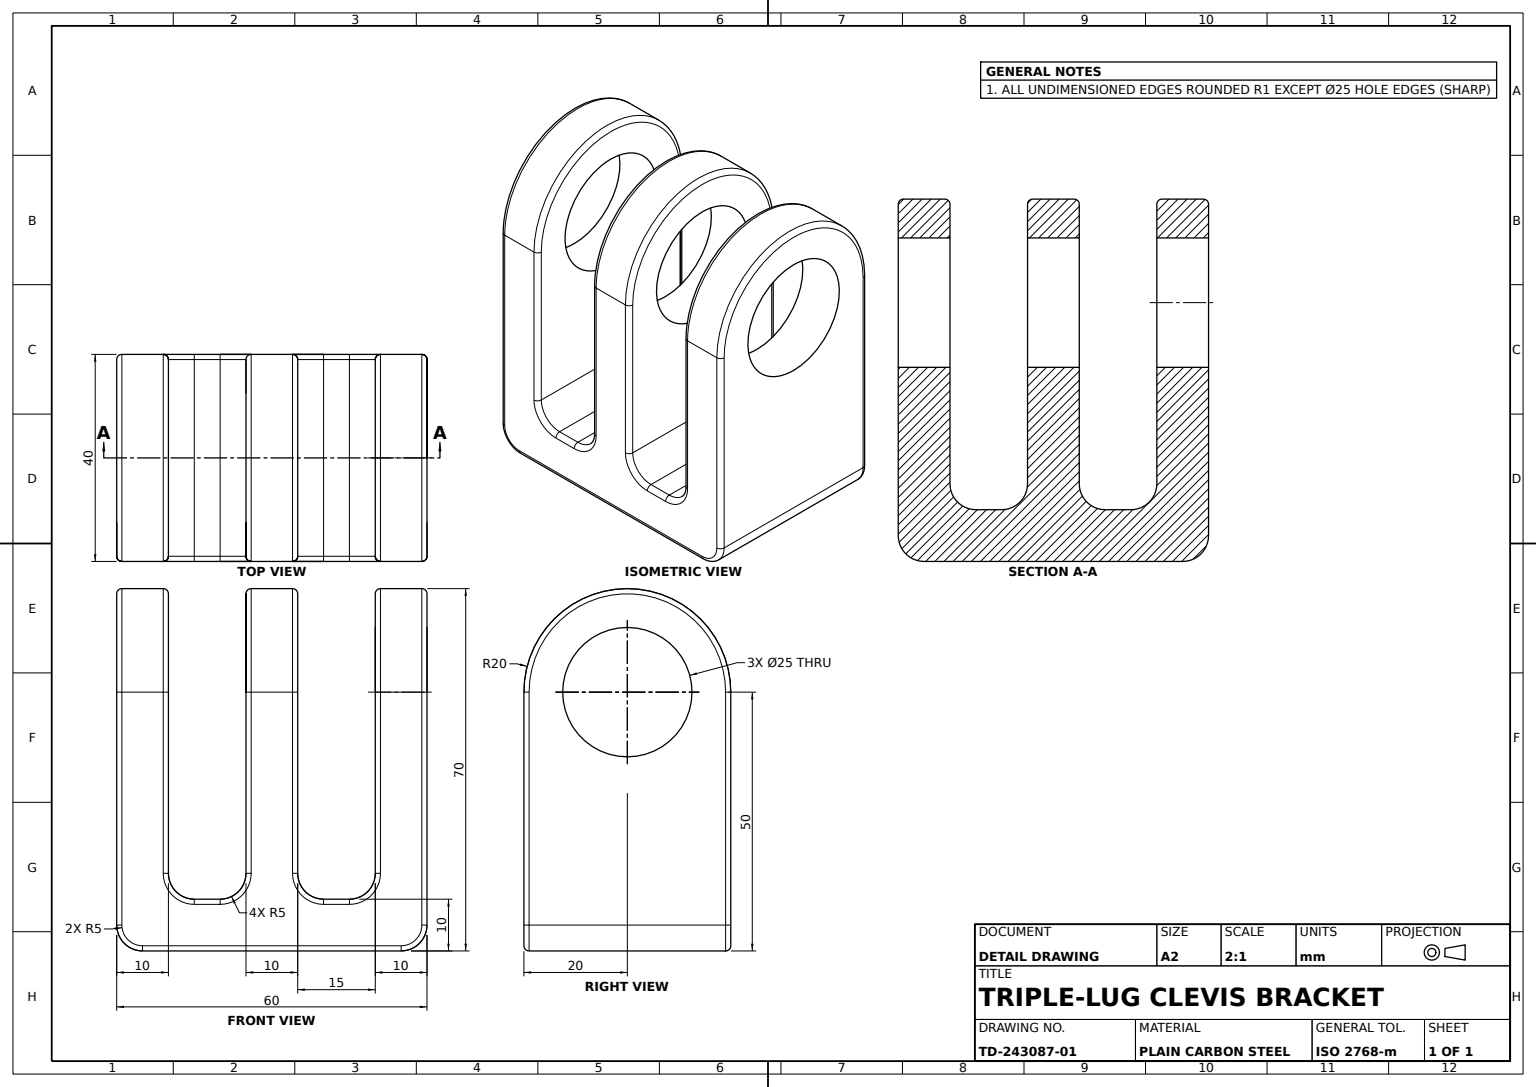
solid
v1 (26,15,20)
v2 (20,9,20)
e1 v1 v2 CIRCLE(AX(P(20,15,20),D(0,0,-1),D(1,0,0)),6)
v3 (25,15,19)
e2 v3 v1 CIRCLE(AX(P(26,15,19),D(0,1,0),D(0,0,1)),1)
v4 (20,10,19)
e3 v4 v3 CIRCLE(AX(P(20,15,19),D(0,0,1),D(1,0,0)),5)
e4 v4 v2 CIRCLE(AX(P(20,9,19),D(1,0,0),D(0,0,-1)),1)
face TORUS(AX(P(20,15,19),D(0,0,1),D(1,0,0)),6,1) [-e1 -e2 -e3 e4]
v5 (35,15,-19)
v6 (34,15,-20)
e5 v5 v6 CIRCLE(AX(P(34,15,-19),D(0,1,0),D(0,0,1)),1)
v7 (40,10,-19)
e6 v7 v5 CIRCLE(AX(P(40,15,-19),D(0,0,-1),D(1,0,0)),5)
v8 (40,9,-20)
e7 v7 v8 CIRCLE(AX(P(40,9,-19),D(-1,0,0),D(0,0,1)),1)
e8 v6 v8 CIRCLE(AX(P(40,15,-20),D(0,0,1),D(1,0,0)),6)
face TORUS(AX(P(40,15,-19),D(0,0,1),D(1,0,0)),6,1) [-e5 -e6 e7 -e8]
v9 (45,10,19)
v10 (45,10,-19)
e9 v9 v10 LINE
e10 v10 v7 LINE
v11 (40,10,19)
e11 v7 v11 LINE
e12 v11 v9 LINE
face PLANE(AX(P(60,10,20),D(0,-1,0),D(1,0,0))) rev [e9 e10 e11 e12]
v12 (40,9,20)
v13 (34,15,20)
e13 v12 v13 CIRCLE(AX(P(40,15,20),D(0,0,-1),D(1,0,0)),6)
e14 v12 v11 CIRCLE(AX(P(40,9,19),D(-1,0,0),D(0,0,1)),1)
v14 (35,15,19)
e15 v14 v11 CIRCLE(AX(P(40,15,19),D(0,0,1),D(1,0,0)),5)
e16 v13 v14 CIRCLE(AX(P(34,15,19),D(0,1,0),D(0,0,1)),1)
face TORUS(AX(P(40,15,19),D(0,0,1),D(1,0,0)),6,1) [-e13 e14 -e15 -e16]
v15 (45,9,-20)
v16 (51,15,-20)
e17 v15 v16 CIRCLE(AX(P(45,15,-20),D(0,0,1),D(1,0,0)),6)
e18 v10 v15 CIRCLE(AX(P(45,9,-19),D(-1,0,0),D(0,0,1)),1)
v17 (50,15,-19)
e19 v17 v10 CIRCLE(AX(P(45,15,-19),D(0,0,-1),D(1,0,0)),5)
e20 v17 v16 CIRCLE(AX(P(51,15,-19),D(0,-1,0),D(0,0,-1)),1)
face TORUS(AX(P(45,15,-19),D(0,0,1),D(1,0,0)),6,1) [-e17 -e18 -e19 e20]
v18 (59,50,-20)
v19 (59,5,-20)
e21 v18 v19 LINE
v20 (60,50,-19)
e22 v18 v20 CIRCLE(AX(P(59,50,-19),D(0,-1,0),D(0,0,-1)),1)
v21 (60,5,-19)
e23 v21 v20 LINE
e24 v19 v21 CIRCLE(AX(P(59,5,-19),D(0,-1,0),D(0,0,-1)),1)
face CYL(AX(P(59,0,-19),D(0,1,0),D(0,0,1)),1) [-e21 e22 -e23 -e24]
v22 (34,50,-20)
e25 v22 v6 LINE
v23 (35,50,-19)
e26 v22 v23 CIRCLE(AX(P(34,50,-19),D(0,-1,0),D(0,0,-1)),1)
e27 v5 v23 LINE
face CYL(AX(P(34,50,-19),D(0,-1,0),D(1,0,0)),1) [e5 -e25 e26 -e27]
v24 (60,5,19)
v25 (59,5,20)
e28 v24 v25 CIRCLE(AX(P(59,5,19),D(0,-1,0),D(0,0,-1)),1)
v26 (60,50,19)
e29 v26 v24 LINE
v27 (59,50,20)
e30 v26 v27 CIRCLE(AX(P(59,50,19),D(0,-1,0),D(0,0,-1)),1)
e31 v25 v27 LINE
face CYL(AX(P(59,0,19),D(0,-1,0),D(0,0,-1)),1) [-e28 -e29 e30 -e31]
v28 (10,37.5,0)
v29 (0,37.5,0)
e32 v28 v29 LINE
v30 (0,62.5,0)
e33 v29 v30 CIRCLE(AX(P(0,50,0),D(-1,0,0),D(0,-1,0)),12.5)
v31 (10,62.5,0)
e34 v31 v30 LINE
e35 v28 v31 CIRCLE(AX(P(10,50,0),D(-1,0,0),D(0,-1,0)),12.5)
face CYL(AX(P(10,50,0),D(-1,0,0),D(0,-1,0)),12.5) rev [e32 e33 -e34 -e35]
v32 (50,15,19)
e36 v9 v32 CIRCLE(AX(P(45,15,19),D(0,0,1),D(1,0,0)),5)
e37 v17 v32 LINE
face CYL(AX(P(45,15,0),D(0,0,-1),D(-1,0,0)),5) rev [e19 -e9 e36 -e37]
v33 (20,10,-19)
v34 (15,10,-19)
e38 v33 v34 LINE
v35 (15,10,19)
e39 v34 v35 LINE
e40 v35 v4 LINE
e41 v4 v33 LINE
face PLANE(AX(P(60,10,20),D(0,-1,0),D(1,0,0))) rev [e38 e39 e40 e41]
v36 (26,70,0)
v37 (26,50,20)
e42 v36 v37 CIRCLE(AX(P(26,50,0),D(1,0,0),D(0,1,0)),20)
v38 (34,50,20)
e43 v38 v37 LINE
v39 (34,70,0)
e44 v38 v39 CIRCLE(AX(P(34,50,0),D(-1,0,0),D(0,1,0)),20)
e45 v39 v22 CIRCLE(AX(P(34,50,0),D(-1,0,0),D(0,1,0)),20)
v40 (26,50,-20)
e46 v22 v40 LINE
e47 v40 v36 CIRCLE(AX(P(26,50,0),D(1,0,0),D(0,1,0)),20)
face CYL(AX(P(35,50,0),D(-1,0,0),D(0,-1,0)),20) [e42 -e43 e44 e45 e46 e47]
v41 (50,50,19)
v42 (50,69,0)
e48 v41 v42 CIRCLE(AX(P(50,50,0),D(-1,0,0),D(0,1,0)),19)
v43 (51,50,20)
e49 v41 v43 CIRCLE(AX(P(51,50,19),D(0,1,0),D(0,0,1)),1)
v44 (51,70,0)
e50 v44 v43 CIRCLE(AX(P(51,50,0),D(1,0,0),D(0,1,0)),20)
e51 v42 v44 CIRCLE(AX(P(51,69,0),D(0,0,-1),D(-1,0,0)),1)
face TORUS(AX(P(51,50,0),D(1,0,0),D(0,1,0)),19,1) [-e48 e49 -e50 -e51]
v45 (5,1,-20)
v46 (1,5,-20)
e52 v45 v46 CIRCLE(AX(P(5,5,-20),D(0,0,-1),D(1,0,0)),4)
v47 (5,0,-19)
e53 v45 v47 CIRCLE(AX(P(5,1,-19),D(-1,0,0),D(0,0,1)),1)
v48 (0,5,-19)
e54 v48 v47 CIRCLE(AX(P(5,5,-19),D(0,0,1),D(1,0,0)),5)
e55 v46 v48 CIRCLE(AX(P(1,5,-19),D(0,1,0),D(0,0,1)),1)
face TORUS(AX(P(5,5,-19),D(0,0,1),D(1,0,0)),4,1) [-e52 e53 -e54 -e55]
v49 (35,69,0)
v50 (35,50,19)
e56 v49 v50 CIRCLE(AX(P(35,50,0),D(1,0,0),D(0,1,0)),19)
e57 v39 v49 CIRCLE(AX(P(34,69,0),D(0,0,-1),D(-1,0,0)),1)
e58 v38 v50 CIRCLE(AX(P(34,50,19),D(0,1,0),D(0,0,1)),1)
face TORUS(AX(P(34,50,0),D(1,0,0),D(0,1,0)),19,1) [-e56 -e57 -e44 e58]
v51 (55,1,20)
e59 v51 v25 CIRCLE(AX(P(55,5,20),D(0,0,1),D(1,0,0)),4)
v52 (55,0,19)
e60 v52 v51 CIRCLE(AX(P(55,1,19),D(-1,0,0),D(0,0,1)),1)
e61 v24 v52 CIRCLE(AX(P(55,5,19),D(0,0,-1),D(1,0,0)),5)
face TORUS(AX(P(55,5,19),D(0,0,1),D(1,0,0)),4,1) [e28 -e59 -e60 -e61]
e62 v14 v5 LINE
face CYL(AX(P(40,15,0),D(0,0,-1),D(-1,0,0)),5) rev [-e11 e6 -e62 e15]
v53 (26,15,-20)
v54 (25,15,-19)
e63 v53 v54 CIRCLE(AX(P(26,15,-19),D(0,1,0),D(0,0,1)),1)
v55 (25,50,-19)
e64 v55 v54 LINE
e65 v55 v40 CIRCLE(AX(P(26,50,-19),D(0,-1,0),D(0,0,-1)),1)
e66 v53 v40 LINE
face CYL(AX(P(26,0,-19),D(0,1,0),D(-1,0,0)),1) [e63 -e64 e65 -e66]
v56 (50,37.5,0)
v57 (50,62.5,0)
e67 v56 v57 CIRCLE(AX(P(50,50,0),D(1,0,0),D(0,1,0)),12.5)
e68 v57 v56 CIRCLE(AX(P(50,50,0),D(1,0,0),D(0,1,0)),12.5)
e69 v32 v41 LINE
v58 (50,50,-19)
e70 v42 v58 CIRCLE(AX(P(50,50,0),D(-1,0,0),D(0,1,0)),19)
e71 v58 v17 LINE
face PLANE(AX(P(50,50,0),D(1,0,0),D(0,1,0))) rev [e67 e68] [e37 e69 e48 e70 e71]
e72 v50 v14 LINE
e73 v13 v38 LINE
face CYL(AX(P(34,50,19),D(0,-1,0),D(1,0,0)),1) [-e72 -e58 -e73 e16]
v59 (51,15,20)
e74 v59 v32 CIRCLE(AX(P(51,15,19),D(0,-1,0),D(0,0,-1)),1)
v60 (45,9,20)
e75 v60 v9 CIRCLE(AX(P(45,9,19),D(-1,0,0),D(0,0,1)),1)
e76 v59 v60 CIRCLE(AX(P(45,15,20),D(0,0,-1),D(1,0,0)),6)
face TORUS(AX(P(45,15,19),D(0,0,1),D(1,0,0)),6,1) [e74 -e36 -e75 -e76]
v61 (25,50,19)
e77 v3 v61 LINE
v62 (25,69,0)
e78 v61 v62 CIRCLE(AX(P(25,50,0),D(-1,0,0),D(0,1,0)),19)
e79 v62 v55 CIRCLE(AX(P(25,50,0),D(-1,0,0),D(0,1,0)),19)
e80 v54 v3 LINE
v63 (25,62.5,0)
v64 (25,37.5,0)
e81 v63 v64 CIRCLE(AX(P(25,50,0),D(1,0,0),D(0,1,0)),12.5)
e82 v64 v63 CIRCLE(AX(P(25,50,0),D(1,0,0),D(0,1,0)),12.5)
face PLANE(AX(P(25,50,0),D(1,0,0),D(0,1,0))) rev [e77 e78 e79 e64 e80] [e81 e82]
v65 (15,9,20)
e83 v35 v65 CIRCLE(AX(P(15,9,19),D(1,0,0),D(0,0,-1)),1)
e84 v2 v65 LINE
face CYL(AX(P(0,9,19),D(1,0,0),D(0,1,0)),1) [-e4 -e40 e83 -e84]
e85 v54 v33 CIRCLE(AX(P(20,15,-19),D(0,0,-1),D(1,0,0)),5)
face CYL(AX(P(20,15,0),D(0,0,-1),D(-1,0,0)),5) rev [-e41 e3 -e80 e85]
v66 (55,0,-19)
e86 v66 v21 CIRCLE(AX(P(55,5,-19),D(0,0,1),D(1,0,0)),5)
v67 (55,1,-20)
e87 v67 v66 CIRCLE(AX(P(55,1,-19),D(-1,0,0),D(0,0,1)),1)
e88 v19 v67 CIRCLE(AX(P(55,5,-20),D(0,0,-1),D(1,0,0)),4)
face TORUS(AX(P(55,5,-19),D(0,0,1),D(1,0,0)),4,1) [e24 -e86 -e87 -e88]
v68 (9,70,0)
v69 (10,69,0)
e89 v68 v69 CIRCLE(AX(P(9,69,0),D(0,0,-1),D(-1,0,0)),1)
v70 (10,50,-19)
e90 v70 v69 CIRCLE(AX(P(10,50,0),D(1,0,0),D(0,1,0)),19)
v71 (9,50,-20)
e91 v71 v70 CIRCLE(AX(P(9,50,-19),D(0,-1,0),D(0,0,-1)),1)
e92 v68 v71 CIRCLE(AX(P(9,50,0),D(-1,0,0),D(0,1,0)),20)
face TORUS(AX(P(9,50,0),D(1,0,0),D(0,1,0)),19,1) [e89 -e90 -e91 -e92]
v72 (9,15,20)
e93 v65 v72 CIRCLE(AX(P(15,15,20),D(0,0,-1),D(1,0,0)),6)
v73 (9,50,20)
e94 v72 v73 LINE
v74 (1,50,20)
e95 v73 v74 LINE
v75 (1,5,20)
e96 v74 v75 LINE
v76 (5,1,20)
e97 v75 v76 CIRCLE(AX(P(5,5,20),D(0,0,1),D(1,0,0)),4)
e98 v76 v51 LINE
e99 v27 v43 LINE
e100 v43 v59 LINE
e101 v60 v12 LINE
e102 v37 v1 LINE
face PLANE(AX(P(0,0,20),D(0,0,1),D(1,0,0))) [e84 e93 e94 e95 e96 e97 e98 e59 e31 e99 e100 e76 e101 e13 e73 e43 e102 e1]
v77 (35,37.5,0)
e103 v77 v64 LINE
v78 (35,62.5,0)
e104 v77 v78 CIRCLE(AX(P(35,50,0),D(1,0,0),D(0,1,0)),12.5)
e105 v78 v63 LINE
face CYL(AX(P(35,50,0),D(-1,0,0),D(0,-1,0)),12.5) rev [-e103 e104 e105 -e82]
v79 (1,50,-20)
e106 v71 v79 LINE
v80 (1,70,0)
e107 v79 v80 CIRCLE(AX(P(1,50,0),D(1,0,0),D(0,1,0)),20)
e108 v80 v74 CIRCLE(AX(P(1,50,0),D(1,0,0),D(0,1,0)),20)
e109 v73 v68 CIRCLE(AX(P(9,50,0),D(-1,0,0),D(0,1,0)),20)
face CYL(AX(P(10,50,0),D(-1,0,0),D(0,-1,0)),20) [e106 e107 e108 -e95 e109 e92]
v81 (0,69,0)
e110 v81 v80 CIRCLE(AX(P(1,69,0),D(0,0,-1),D(-1,0,0)),1)
v82 (0,50,19)
e111 v82 v81 CIRCLE(AX(P(0,50,0),D(-1,0,0),D(0,1,0)),19)
e112 v82 v74 CIRCLE(AX(P(1,50,19),D(0,1,0),D(0,0,1)),1)
face TORUS(AX(P(1,50,0),D(1,0,0),D(0,1,0)),19,1) [-e108 -e110 -e111 e112]
e113 v66 v52 LINE
v83 (5,0,19)
e114 v52 v83 LINE
e115 v83 v47 LINE
e116 v47 v66 LINE
face PLANE(AX(P(0,0,20),D(0,1,0),D(0,0,1))) rev [e113 e114 e115 e116]
v84 (0,5,19)
e117 v84 v82 LINE
e118 v84 v75 CIRCLE(AX(P(1,5,19),D(0,1,0),D(0,0,1)),1)
face CYL(AX(P(1,0,19),D(0,1,0),D(-1,0,0)),1) [-e112 -e117 e118 -e96]
v85 (0,50,-19)
e119 v85 v48 LINE
e120 v79 v85 CIRCLE(AX(P(1,50,-19),D(0,1,0),D(0,0,1)),1)
e121 v46 v79 LINE
face CYL(AX(P(1,10,-19),D(0,-1,0),D(1,0,0)),1) [-e119 -e120 -e121 e55]
e122 v20 v26 CIRCLE(AX(P(60,50,0),D(1,0,0),D(0,0,1)),19)
e123 v27 v18 CIRCLE(AX(P(59,50,0),D(-1,0,0),D(0,0,1)),20)
face TORUS(AX(P(59,50,0),D(-1,0,0),D(0,0,1)),19,1) [-e30 -e122 -e22 -e123]
e124 v61 v37 CIRCLE(AX(P(26,50,19),D(0,1,0),D(0,0,1)),1)
e125 v62 v36 CIRCLE(AX(P(26,69,0),D(0,0,-1),D(-1,0,0)),1)
face TORUS(AX(P(26,50,0),D(1,0,0),D(0,1,0)),19,1) [e124 -e42 -e125 -e78]
e126 v83 v84 CIRCLE(AX(P(5,5,19),D(0,0,-1),D(1,0,0)),5)
e127 v48 v84 LINE
face CYL(AX(P(5,5,20),D(0,0,1),D(1,0,0)),5) [e126 -e127 e54 -e115]
e128 v83 v76 CIRCLE(AX(P(5,1,19),D(-1,0,0),D(0,0,1)),1)
face TORUS(AX(P(5,5,19),D(0,0,1),D(1,0,0)),4,1) [-e118 -e126 e128 -e97]
e129 v78 v77 CIRCLE(AX(P(35,50,0),D(1,0,0),D(0,1,0)),12.5)
face CYL(AX(P(35,50,0),D(-1,0,0),D(0,-1,0)),12.5) rev [e103 -e81 -e105 e129]
face CYL(AX(P(0,9,19),D(1,0,0),D(0,1,0)),1) [e75 -e12 -e14 -e101]
e130 v24 v21 LINE
face CYL(AX(P(55,5,20),D(0,0,-1),D(-1,0,0)),5) [e61 -e113 e86 -e130]
face CYL(AX(P(26,0,19),D(0,1,0),D(-1,0,0)),1) [e2 -e102 -e124 -e77]
v86 (60,37.5,0)
e131 v86 v56 LINE
v87 (60,62.5,0)
e132 v86 v87 CIRCLE(AX(P(60,50,0),D(1,0,0),D(0,1,0)),12.5)
e133 v87 v57 LINE
face CYL(AX(P(60,50,0),D(-1,0,0),D(0,-1,0)),12.5) rev [-e67 -e131 e132 e133]
e134 v87 v86 CIRCLE(AX(P(60,50,0),D(1,0,0),D(0,1,0)),12.5)
face PLANE(AX(P(60,0,20),D(-1,0,0),D(0,0,1))) rev [-e132 -e134] [e29 e130 e23 e122]
v88 (51,50,-20)
e135 v58 v88 CIRCLE(AX(P(51,50,-19),D(0,-1,0),D(0,0,-1)),1)
e136 v16 v88 LINE
face CYL(AX(P(51,0,-19),D(0,1,0),D(-1,0,0)),1) [e135 -e136 -e20 -e71]
face TORUS(AX(P(26,50,0),D(1,0,0),D(0,1,0)),19,1) [-e79 e125 -e47 -e65]
v89 (10,15,19)
e137 v89 v35 CIRCLE(AX(P(15,15,19),D(0,0,1),D(1,0,0)),5)
e138 v89 v72 CIRCLE(AX(P(9,15,19),D(0,-1,0),D(0,0,-1)),1)
face TORUS(AX(P(15,15,19),D(0,0,1),D(1,0,0)),6,1) [-e137 e138 -e93 -e83]
e139 v88 v44 CIRCLE(AX(P(51,50,0),D(1,0,0),D(0,1,0)),20)
face TORUS(AX(P(51,50,0),D(1,0,0),D(0,1,0)),19,1) [-e70 e51 -e139 -e135]
v90 (9,15,-20)
e140 v71 v90 LINE
v91 (10,15,-19)
e141 v91 v70 LINE
e142 v90 v91 CIRCLE(AX(P(9,15,-19),D(0,-1,0),D(0,0,-1)),1)
face CYL(AX(P(9,0,-19),D(0,1,0),D(-1,0,0)),1) [-e140 e91 -e141 -e142]
e143 v67 v45 LINE
face CYL(AX(P(0,1,-19),D(1,0,0),D(0,0,-1)),1) [-e143 e87 -e116 -e53]
e144 v23 v49 CIRCLE(AX(P(35,50,0),D(1,0,0),D(0,1,0)),19)
face TORUS(AX(P(34,50,0),D(1,0,0),D(0,1,0)),19,1) [-e45 e57 -e144 -e26]
face CYL(AX(P(60,50,0),D(-1,0,0),D(0,-1,0)),12.5) rev [-e133 e134 e131 -e68]
e145 v18 v88 LINE
v92 (15,9,-20)
e146 v90 v92 CIRCLE(AX(P(15,15,-20),D(0,0,1),D(1,0,0)),6)
v93 (20,9,-20)
e147 v92 v93 LINE
e148 v93 v53 CIRCLE(AX(P(20,15,-20),D(0,0,1),D(1,0,0)),6)
e149 v8 v15 LINE
face PLANE(AX(P(0,0,-20),D(0,0,1),D(1,0,0))) rev [e136 -e145 e21 e88 e143 e52 e121 -e106 e140 e146 e147 e148 e66 -e46 e25 e8 e149 e17]
face CYL(AX(P(0,1,19),D(-1,0,0),D(0,0,1)),1) [e60 -e98 -e128 -e114]
v94 (10,50,19)
e150 v73 v94 CIRCLE(AX(P(9,50,19),D(0,1,0),D(0,0,1)),1)
e151 v69 v94 CIRCLE(AX(P(10,50,0),D(1,0,0),D(0,1,0)),19)
face TORUS(AX(P(9,50,0),D(1,0,0),D(0,1,0)),19,1) [-e89 -e109 e150 -e151]
face CYL(AX(P(51,0,19),D(0,1,0),D(-1,0,0)),1) [-e100 -e49 -e69 -e74]
e152 v81 v85 CIRCLE(AX(P(0,50,0),D(-1,0,0),D(0,1,0)),19)
face TORUS(AX(P(1,50,0),D(1,0,0),D(0,1,0)),19,1) [-e107 e120 -e152 e110]
e153 v92 v34 CIRCLE(AX(P(15,9,-19),D(1,0,0),D(0,0,-1)),1)
e154 v93 v33 CIRCLE(AX(P(20,9,-19),D(1,0,0),D(0,0,-1)),1)
face CYL(AX(P(60,9,-19),D(-1,0,0),D(0,-1,0)),1) [-e147 e153 -e38 -e154]
e155 v30 v29 CIRCLE(AX(P(0,50,0),D(-1,0,0),D(0,-1,0)),12.5)
face PLANE(AX(P(0,10,20),D(1,0,0),D(0,1,0))) rev [-e155 -e33] [e127 e117 e111 e152 e119]
e156 v94 v89 LINE
face CYL(AX(P(9,0,19),D(0,1,0),D(-1,0,0)),1) [-e94 -e138 -e156 -e150]
e157 v89 v91 LINE
e158 v31 v28 CIRCLE(AX(P(10,50,0),D(-1,0,0),D(0,-1,0)),12.5)
face PLANE(AX(P(10,50,0),D(1,0,0),D(0,1,0))) [e156 e157 e141 e90 e151] [e158 e35]
face PLANE(AX(P(35,50,0),D(1,0,0),D(0,1,0))) [e62 e27 e144 e56 e72] [-e104 -e129]
e159 v34 v91 CIRCLE(AX(P(15,15,-19),D(0,0,-1),D(1,0,0)),5)
face TORUS(AX(P(15,15,-19),D(0,0,1),D(1,0,0)),6,1) [-e159 -e153 -e146 e142]
face CYL(AX(P(10,50,0),D(-1,0,0),D(0,-1,0)),12.5) rev [-e32 -e158 e34 e155]
face TORUS(AX(P(20,15,-19),D(0,0,1),D(1,0,0)),6,1) [e154 -e85 -e63 -e148]
face CYL(AX(P(60,50,0),D(-1,0,0),D(0,-1,0)),20) [e123 e145 e139 e50 -e99]
face CYL(AX(P(60,9,-19),D(-1,0,0),D(0,-1,0)),1) [-e149 -e7 -e10 e18]
face CYL(AX(P(15,15,0),D(0,0,-1),D(-1,0,0)),5) rev [-e157 e137 -e39 e159]
